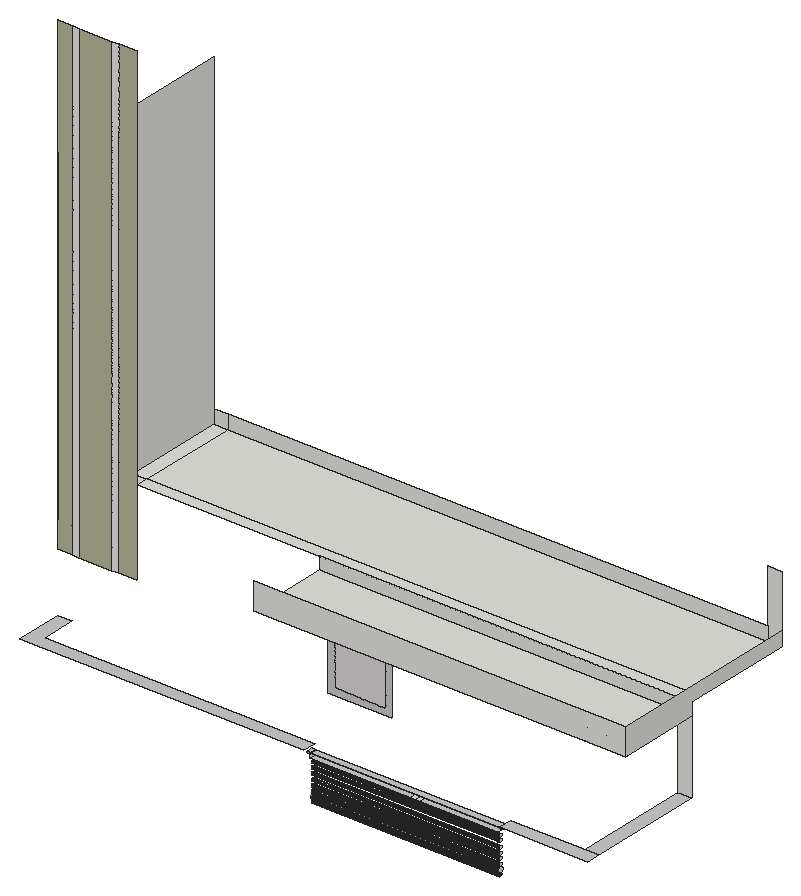
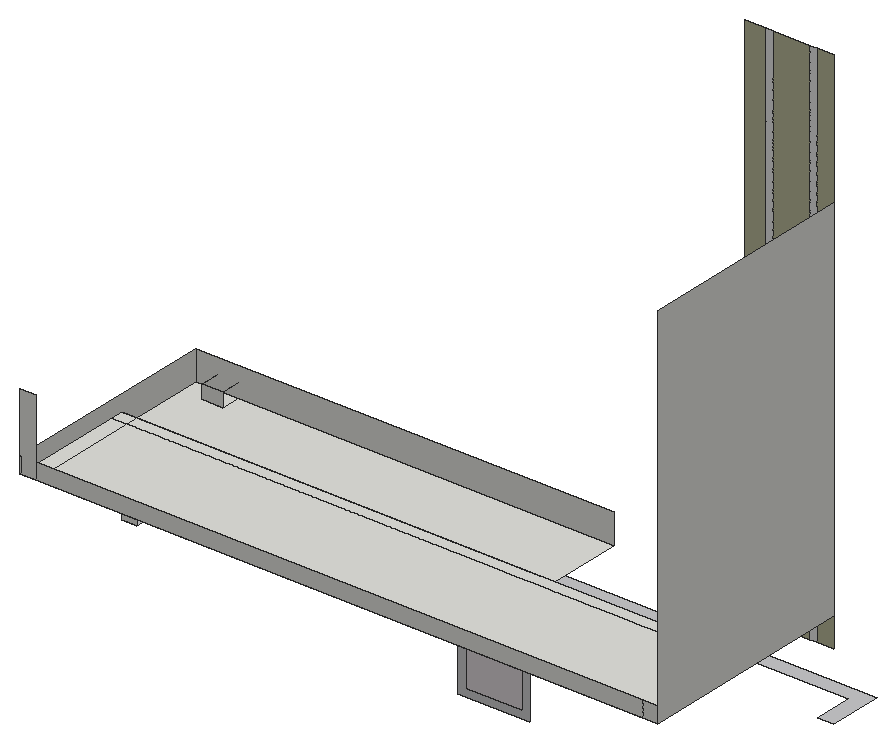
# SketchUp Ruby script. Lengths in inches.
U = 1.inch
M = Sketchup.active_model
def pt(a) = Geom::Point3d.new(a.map { |v| v * U })
def face(e, loops, mat)
  f = e.add_face(loops[0].map { |a| pt(a) })
  loops[1..].each { |l| e.add_face(l.map { |a| pt(a) }).erase! }
  f.material = f.back_material = mat if mat
  f
end
# faces: each face lists its corners as indices into pts; further lists are holes
def faces(e, pts, list, mat = nil) = list.each { |f| face(e, (f[0].is_a?(Array) ? f : [f]).map { |l| l.map { |i| pts[i] } }, mat) }
# xy, xz, yz: faces in a plane at the given z, y or x. An outline is a flat list of corners, or four numbers for a rectangle; further outlines are holes
def ring(l) = l.size == 4 ? [[l[0], l[1]], [l[2], l[1]], [l[2], l[3]], [l[0], l[3]]] : l.each_slice(2).to_a
def flat(e, list, mat, &to3) = list.each { |f| face(e, (f[0].is_a?(Array) ? f : [f]).map { |l| ring(l).map { |u, v| to3.(u, v) } }, mat) }
def xy(e, z, list, mat = nil) = flat(e, list, mat) { |x, y| [x, y, z] }
def xz(e, y, list, mat = nil) = flat(e, list, mat) { |x, z| [x, y, z] }
def yz(e, x, list, mat = nil) = flat(e, list, mat) { |y, z| [x, y, z] }
def lines(e, pts, list) = list.each { |a, b| e.add_line(pt(pts[a]), pt(pts[b])) }
# prism: a flat outline (further loops are holes) pulled along v
def prism(e, loops, v, mat = nil)
  f = face(e, loops, mat); d = Geom::Vector3d.new(v.map { |x| x * U })
  f.pushpull(f.normal.samedirection?(d) ? d.length : -d.length)
end
def box(e, o, s, mat = nil) = prism(e, [[o, [o[0] + s[0], o[1], o[2]], [o[0] + s[0], o[1] + s[1], o[2]], [o[0], o[1] + s[1], o[2]]]], [0, 0, s[2]], mat)
def at(x, y, z, deg = 0) = Geom::Transformation.translation(pt([x, y, z])) * Geom::Transformation.rotation(ORIGIN, Z_AXIS, deg.degrees)
def axes(o, x, y, z) = Geom::Transformation.new([*x, 0, *y, 0, *z, 0, *pt(o).to_a, 1])
def part(name) = M.definitions.add(name)
# library, detail: a bought-in or finely detailed component or shape, given as its bounding box
def library(name, o, s) = part(name).tap { |d| box(d.entities, o, s) }
def detail(e, o, s) = box(e.add_group.entities, o, s)
def put(e, d, t, mat = nil) = e.add_instance(d, t).tap { |i| i.material = mat if mat }
def group(e, t, mat = nil) = e.add_group.tap { |g| g.transformation = t; g.material = mat if mat }.entities
root = M.entities
M.materials.add("[Blinds Cellular White]").color = [217, 211, 213]
M.materials.add("[Concrete Form 4x8]").color = [167, 170, 168]
M.materials.add("[Polished Concrete New]").color = [200, 200, 203]
M.materials.add("[Polished Concrete Old]").color = [229, 229, 229]
M.materials.add("[Tile Linen]").color = [182, 181, 151]
xy(root,149.47,[[768.81,230.26,772.74,230.26,772.74,243.6875,764.33,243.6875,764.33,230.27],[754.67,230.27,764.33,243.6875],[754.67,243.6875,764.33,243.6875,764.33,243.85,754.67,243.86],[764.33,243.6875,772.74,243.6875,772.74,243.84,768.82,243.84,764.33,243.85]])
xy(root,149.47,[[562.43,230.1,562.43,243.6875,754.67,243.6875,754.67,230.27,764.33,230.27,768.81,230.26,772.74,230.26,772.74,243.6875,922.51,243.6875,922.51,230.1]],"[Polished Concrete New]")
xy(root,158.26,[[562.43,230.1,931.07,243.6875],[555.05,230.47,562.43,244.05]],"[Polished Concrete New]")
xy(root,163.5625,[[11.875,223.5,555.05,223.5,555.05,249.9,38.27,249.9,38.27,314.12,11.875,314.12],[931.07,223.5,1099.23,249.9],[1072.84,249.9,1099.23,472.99]],"[Polished Concrete New]")
xy(root,304.3125,[[386.67,314.12,386.67,472.99,1099.23,472.99,1099.23,314.12,1062.63,314.12,1062.63,346.6,1027.11,346.6,1027.11,314.12],[1027.11,314.12,1062.63,346.6]])
xy(root,328.125,[[11.875,472.99,38.27,494.96],[38.27,472.99,1072.84,494.96],[1072.84,472.99,1099.23,494.96],[11.875,494.96,38.27,688.57],[38.27,494.96,1072.84,688.57],
  [1072.84,494.96,1099.23,688.57]])
xz(root,230.1,[[562.43,158,931.07,158.26]])
xz(root,230.47,[[555.05,158,562.43,158.26]])
xz(root,314.12,[[386.67,304.3125,1099.23,354.875]])
xz(root,314.12,[[40.46,278.16,52.5,1185.41],[116.02,278.16,128.0625,1185.41]],"[Polished Concrete Old]")
xz(root,314.12,[[11.875,278.16,40.46,1185.41],[52.5,278.16,116.02,1185.41],[128.0625,278.16,163.125,1185.41]],"[Tile Linen]")
xz(root,346.6,[[1027.11,304.3125,1062.63,328.125]])
xz(root,472.99,[[1072.84,163.5625,1099.23,304.3125],[386.67,304.3125,1072.84,328.125],[1072.84,304.3125,1099.23,328.125]])
xz(root,472.99,[[414.74,111.09,512.86,284.96]],"[Blinds Cellular White]")
xz(root,472.99,[[[402.52,98.87,525.08,297.18],[414.74,111.09,512.86,284.96]]],"[Polished Concrete New]")
xz(root,688.57,[[11.875,328.125,38.27,354.875],[38.27,328.125,1072.84,354.875],[1072.84,328.125,1099.23,457.5]])
yz(root,11.875,[[314.12,328.125,688.57,958.5625]])
yz(root,562.43,[[230.1,149.47,230.47,158.26],[230.47,149.47,243.6875,158.26]])
yz(root,922.51,[[236.62,77.51,237.7,77.65,238.71,78.07,239.58,78.74,240.24,79.6,240.66,80.61,240.81,81.7,240.66,82.78,240.24,83.79,239.58,84.66,238.71,85.32,237.7,85.74,236.62,85.89,235.53,85.74,234.52,85.32,233.66,84.66,232.99,83.79,232.57,82.78,232.43,81.7,232.57,80.61,232.99,79.6,233.66,78.74,234.52,78.07,235.53,77.65],[236.71,89.28,237.35,89.36,237.93,89.61,238.4375,89.99,238.83,90.5,239.07,91.09,239.15,91.72,239.07,92.35,238.83,92.9375,238.4375,93.44,237.93,93.83,237.35,94.07,236.71,94.15,236.08,94.07,235.5,93.83,234.99,93.44,234.6,92.9375,234.36,92.35,234.28,91.72,234.36,91.09,234.6,90.5,234.99,89.99,235.5,89.61,236.08,89.36],[236.71,98.28,237.35,98.36,237.93,98.61,238.4375,98.99,238.83,99.5,239.07,100.09,239.15,100.72,239.07,101.35,238.83,101.9375,238.4375,102.44,237.93,102.83,237.35,103.07,236.71,103.15,236.08,103.07,235.5,102.83,234.99,102.44,234.6,101.9375,234.36,101.35,234.28,100.72,234.36,100.09,234.6,99.5,234.99,98.99,235.5,98.61,236.08,98.36],[236.71,108.15,237.35,108.24,237.93,108.48,238.4375,108.87,238.83,109.375,239.07,109.96,239.15,110.59,239.07,111.22,238.83,111.8125,238.4375,112.32,237.93,112.7,237.35,112.95,236.71,113.03,236.08,112.95,235.5,112.7,234.99,112.32,234.6,111.8125,234.36,111.22,234.28,110.59,234.36,109.96,234.6,109.375,234.99,108.87,235.5,108.48,236.08,108.24],[236.71,118.53,237.35,118.61,237.93,118.86,238.4375,119.24,238.83,119.75,239.07,120.34,239.15,120.97,239.07,121.6,238.83,122.1875,238.4375,122.69,237.93,123.08,237.35,123.32,236.71,123.4,236.08,123.32,235.5,123.08,234.99,122.69,234.6,122.1875,234.36,121.6,234.28,120.97,234.36,120.34,234.6,119.75,234.99,119.24,235.5,118.86,236.08,118.61],
  [236.71,129.34,237.35,129.43,237.93,129.67,238.4375,130.06,238.83,130.5625,239.07,131.15,239.15,131.78,239.07,132.41,238.83,133,238.4375,133.5,237.93,133.89,237.35,134.13,236.71,134.22,236.08,134.13,235.5,133.89,234.99,133.5,234.6,133,234.36,132.41,234.28,131.78,234.36,131.15,234.6,130.5625,234.99,130.06,235.5,129.67,236.08,129.43],[236.71,138.15,237.35,138.24,237.93,138.48,238.4375,138.87,238.83,139.375,239.07,139.96,239.15,140.59,239.07,141.22,238.83,141.8125,238.4375,142.32,237.93,142.7,237.35,142.95,236.71,143.03,236.08,142.95,235.5,142.7,234.99,142.32,234.6,141.8125,234.36,141.22,234.28,140.59,234.36,139.96,234.6,139.375,234.99,138.87,235.5,138.48,236.08,138.24]])
yz(root,1099.23,[[314.12,304.3125,472.99,304.3125,472.99,328.125,688.57,328.125,688.57,354.875,314.12,354.875]])
p = [[922.51,234.6,71.4375],[922.51,234.36,72.02],[562.43,234.36,72.02],[562.43,234.6,71.4375],[922.51,239.07,72.02],[922.51,238.83,71.4375],
  [562.43,238.83,71.4375],[562.43,239.07,72.02],[922.51,234.28,72.65],[562.43,234.28,72.65],[922.51,239.15,72.65],[562.43,239.15,72.65],
  [922.51,234.36,73.29],[562.43,234.36,73.29],[922.51,239.07,73.29],[562.43,239.07,73.29],[922.51,234.6,73.875],[562.43,234.6,73.875],
  [922.51,238.83,73.875],[562.43,238.83,73.875],[922.51,234.99,74.38],[562.43,234.99,74.38],[922.51,238.4375,74.38],[562.43,238.4375,74.38],
  [922.51,235.5,74.77],[562.43,235.5,74.77],[922.51,237.93,74.77],[562.43,237.93,74.77],[922.51,236.08,75.01],[562.43,236.08,75.01],
  [922.51,237.35,75.01],[562.43,237.35,75.01],[922.51,236.71,75.09],[562.43,236.71,75.09],[922.51,236.62,77.51],[922.51,235.53,77.65],
  [562.43,235.53,77.65],[562.43,236.62,77.51],[922.51,237.7,77.65],[562.43,237.7,77.65],[922.51,234.52,78.07],[562.43,234.52,78.07],
  [922.51,238.71,78.07],[562.43,238.71,78.07],[922.51,233.66,78.74],[562.43,233.66,78.74],[922.51,239.58,78.74],[562.43,239.58,78.74],
  [922.51,232.99,79.6],[562.43,232.99,79.6],[922.51,240.24,79.6],[562.43,240.24,79.6],[922.51,232.57,80.61],[562.43,232.57,80.61],
  [922.51,240.66,80.61],[562.43,240.66,80.61],[922.51,232.43,81.7],[562.43,232.43,81.7],[922.51,240.81,81.7],[562.43,240.81,81.7],
  [922.51,232.57,82.78],[562.43,232.57,82.78],[922.51,240.66,82.78],[562.43,240.66,82.78],[922.51,232.99,83.79],[562.43,232.99,83.79],
  [922.51,240.24,83.79],[562.43,240.24,83.79],[922.51,233.66,84.66],[562.43,233.66,84.66],[922.51,239.58,84.66],[562.43,239.58,84.66],
  [922.51,234.52,85.32],[562.43,234.52,85.32],[922.51,238.71,85.32],[562.43,238.71,85.32],[922.51,235.53,85.74],[562.43,235.53,85.74],
  [922.51,237.7,85.74],[562.43,237.7,85.74],[922.51,236.62,85.89],[562.43,236.62,85.89],[922.51,236.71,89.28],[922.51,236.08,89.36],
  [562.43,236.08,89.36],[562.43,236.71,89.28],[922.51,237.35,89.36],[562.43,237.35,89.36],[922.51,235.5,89.61],[562.43,235.5,89.61],
  [922.51,237.93,89.61],[562.43,237.93,89.61],[922.51,234.99,89.99],[562.43,234.99,89.99],[922.51,238.4375,89.99],[562.43,238.4375,89.99],
  [922.51,234.6,90.5],[562.43,234.6,90.5],[922.51,238.83,90.5],[562.43,238.83,90.5],[922.51,234.36,91.09],[562.43,234.36,91.09],
  [922.51,239.07,91.09],[562.43,239.07,91.09],[922.51,234.28,91.72],[562.43,234.28,91.72],[922.51,239.15,91.72],[562.43,239.15,91.72],
  [922.51,234.36,92.35],[562.43,234.36,92.35],[922.51,239.07,92.35],[562.43,239.07,92.35],[922.51,234.6,92.9375],[562.43,234.6,92.9375],
  [922.51,238.83,92.9375],[562.43,238.83,92.9375],[922.51,234.99,93.44],[562.43,234.99,93.44],[922.51,238.4375,93.44],[562.43,238.4375,93.44],
  [922.51,235.5,93.83],[562.43,235.5,93.83],[922.51,237.93,93.83],[562.43,237.93,93.83],[922.51,236.08,94.07],[562.43,236.08,94.07],
  [922.51,237.35,94.07],[562.43,237.35,94.07],[922.51,236.71,94.15],[562.43,236.71,94.15],[922.51,236.71,98.28],[922.51,236.08,98.36],
  [562.43,236.08,98.36],[562.43,236.71,98.28],[922.51,237.35,98.36],[562.43,237.35,98.36],[922.51,235.5,98.61],[562.43,235.5,98.61],
  [922.51,237.93,98.61],[562.43,237.93,98.61],[922.51,234.99,98.99],[562.43,234.99,98.99],[922.51,238.4375,98.99],[562.43,238.4375,98.99],
  [922.51,234.6,99.5],[562.43,234.6,99.5],[922.51,238.83,99.5],[562.43,238.83,99.5],[922.51,234.36,100.09],[562.43,234.36,100.09],
  [922.51,239.07,100.09],[562.43,239.07,100.09],[922.51,234.28,100.72],[562.43,234.28,100.72],[922.51,239.15,100.72],[562.43,239.15,100.72],
  [922.51,234.36,101.35],[562.43,234.36,101.35],[922.51,239.07,101.35],[562.43,239.07,101.35],[922.51,234.6,101.9375],[562.43,234.6,101.9375],
  [922.51,238.83,101.9375],[562.43,238.83,101.9375],[922.51,234.99,102.44],[562.43,234.99,102.44],[922.51,238.4375,102.44],[562.43,238.4375,102.44],
  [922.51,235.5,102.83],[562.43,235.5,102.83],[922.51,237.93,102.83],[562.43,237.93,102.83],[922.51,236.08,103.07],[562.43,236.08,103.07],
  [922.51,237.35,103.07],[562.43,237.35,103.07],[922.51,236.71,103.15],[562.43,236.71,103.15],[922.51,236.08,108.24],[922.51,235.5,108.48],
  [562.43,235.5,108.48],[562.43,236.08,108.24],[922.51,236.71,108.15],[562.43,236.71,108.15],[922.51,237.35,108.24],[562.43,237.35,108.24],
  [922.51,237.93,108.48],[562.43,237.93,108.48],[922.51,234.99,108.87],[562.43,234.99,108.87],[922.51,238.4375,108.87],[562.43,238.4375,108.87],
  [922.51,234.6,109.375],[562.43,234.6,109.375],[922.51,238.83,109.375],[562.43,238.83,109.375],[922.51,234.36,109.96],[562.43,234.36,109.96],
  [922.51,239.07,109.96],[562.43,239.07,109.96],[922.51,234.28,110.59],[562.43,234.28,110.59],[922.51,239.15,110.59],[562.43,239.15,110.59],
  [922.51,234.36,111.22],[562.43,234.36,111.22],[922.51,239.07,111.22],[562.43,239.07,111.22],[922.51,234.6,111.8125],[562.43,234.6,111.8125],
  [922.51,238.83,111.8125],[562.43,238.83,111.8125],[922.51,234.99,112.32],[562.43,234.99,112.32],[922.51,238.4375,112.32],[562.43,238.4375,112.32],
  [922.51,235.5,112.7],[562.43,235.5,112.7],[922.51,237.93,112.7],[562.43,237.93,112.7],[922.51,236.08,112.95],[562.43,236.08,112.95],
  [922.51,237.35,112.95],[562.43,237.35,112.95],[922.51,236.71,113.03],[562.43,236.71,113.03],[922.51,236.71,118.53],[922.51,236.08,118.61],
  [562.43,236.08,118.61],[562.43,236.71,118.53],[922.51,237.35,118.61],[562.43,237.35,118.61],[922.51,235.5,118.86],[562.43,235.5,118.86],
  [922.51,237.93,118.86],[562.43,237.93,118.86],[922.51,234.99,119.24],[562.43,234.99,119.24],[922.51,238.4375,119.24],[562.43,238.4375,119.24],
  [922.51,234.6,119.75],[562.43,234.6,119.75],[922.51,238.83,119.75],[562.43,238.83,119.75],[922.51,234.36,120.34],[562.43,234.36,120.34],
  [922.51,239.07,120.34],[562.43,239.07,120.34],[922.51,234.28,120.97],[562.43,234.28,120.97],[922.51,239.15,120.97],[562.43,239.15,120.97],
  [922.51,234.36,121.6],[562.43,234.36,121.6],[922.51,239.07,121.6],[562.43,239.07,121.6],[922.51,234.6,122.1875],[562.43,234.6,122.1875],
  [922.51,238.83,122.1875],[562.43,238.83,122.1875],[922.51,234.99,122.69],[562.43,234.99,122.69],[922.51,238.4375,122.69],[562.43,238.4375,122.69],
  [922.51,235.5,123.08],[562.43,235.5,123.08],[922.51,237.93,123.08],[562.43,237.93,123.08],[922.51,236.08,123.32],[562.43,236.08,123.32],
  [922.51,237.35,123.32],[562.43,237.35,123.32],[922.51,236.71,123.4],[562.43,236.71,123.4],[922.51,236.71,129.34],[922.51,236.08,129.43],
  [562.43,236.08,129.43],[562.43,236.71,129.34],[922.51,237.35,129.43],[562.43,237.35,129.43],[922.51,235.5,129.67],[562.43,235.5,129.67],
  [922.51,237.93,129.67],[562.43,237.93,129.67],[922.51,234.99,130.06],[562.43,234.99,130.06],[922.51,238.4375,130.06],[562.43,238.4375,130.06],
  [922.51,234.6,130.5625],[562.43,234.6,130.5625],[922.51,238.83,130.5625],[562.43,238.83,130.5625],[922.51,234.36,131.15],[562.43,234.36,131.15],
  [922.51,239.07,131.15],[562.43,239.07,131.15],[922.51,234.28,131.78],[562.43,234.28,131.78],[922.51,239.15,131.78],[562.43,239.15,131.78],
  [922.51,234.36,132.41],[562.43,234.36,132.41],[922.51,239.07,132.41],[562.43,239.07,132.41],[922.51,234.6,133],[562.43,234.6,133],
  [922.51,238.83,133],[562.43,238.83,133],[922.51,234.99,133.5],[562.43,234.99,133.5],[922.51,238.4375,133.5],[562.43,238.4375,133.5],
  [922.51,235.5,133.89],[562.43,235.5,133.89],[922.51,237.93,133.89],[562.43,237.93,133.89],[922.51,236.08,134.13],[562.43,236.08,134.13],
  [922.51,237.35,134.13],[562.43,237.35,134.13],[922.51,236.71,134.22],[562.43,236.71,134.22],[922.51,236.08,138.24],[922.51,235.5,138.48],
  [562.43,235.5,138.48],[562.43,236.08,138.24],[922.51,236.71,138.15],[562.43,236.71,138.15],[922.51,237.35,138.24],[562.43,237.35,138.24],
  [922.51,237.93,138.48],[562.43,237.93,138.48],[922.51,234.99,138.87],[562.43,234.99,138.87],[922.51,238.4375,138.87],[562.43,238.4375,138.87],
  [922.51,234.6,139.375],[562.43,234.6,139.375],[922.51,238.83,139.375],[562.43,238.83,139.375],[922.51,234.36,139.96],[562.43,234.36,139.96],
  [922.51,239.07,139.96],[562.43,239.07,139.96],[922.51,234.28,140.59],[562.43,234.28,140.59],[922.51,239.15,140.59],[562.43,239.15,140.59],
  [922.51,234.36,141.22],[562.43,234.36,141.22],[922.51,239.07,141.22],[562.43,239.07,141.22],[922.51,234.6,141.8125],[562.43,234.6,141.8125],
  [922.51,238.83,141.8125],[562.43,238.83,141.8125],[922.51,234.99,142.32],[562.43,234.99,142.32],[922.51,238.4375,142.32],[562.43,238.4375,142.32],
  [922.51,235.5,142.7],[562.43,235.5,142.7],[922.51,237.93,142.7],[562.43,237.93,142.7],[922.51,236.08,142.95],[562.43,236.08,142.95],
  [922.51,237.35,142.95],[562.43,237.35,142.95],[922.51,236.71,143.03],[562.43,236.71,143.03],[1062.63,346.6,328.125],[1062.63,314.12,328.125],
  [1027.11,346.6,328.125],[1027.11,314.12,328.125],[38.27,472.99,328.125],[38.27,314.12,328.125]]
faces(root,p,[[0,1,2,3],[4,5,6,7],[1,8,9,2],[10,4,7,11],[8,12,13,9],[14,10,11,15],[12,16,17,13],[18,14,15,19],
  [16,20,21,17],[22,18,19,23],[20,24,25,21],[26,22,23,27],[24,28,29,25],[30,26,27,31],[28,32,33,29],[32,30,31,33],
  [82,83,84,85],[86,82,85,87],[83,88,89,84],[90,86,87,91],[88,92,93,89],[94,90,91,95],[92,96,97,93],[98,94,95,99],
  [96,100,101,97],[102,98,99,103],[100,104,105,101],[106,102,103,107],[104,108,109,105],[110,106,107,111],[108,112,113,109],[114,110,111,115],
  [112,116,117,113],[118,114,115,119],[116,120,121,117],[122,118,119,123],[120,124,125,121],[126,122,123,127],[124,128,129,125],[128,126,127,129],
  [130,131,132,133],[134,130,133,135],[131,136,137,132],[138,134,135,139],[136,140,141,137],[142,138,139,143],[140,144,145,141],[146,142,143,147],
  [144,148,149,145],[150,146,147,151],[148,152,153,149],[154,150,151,155],[152,156,157,153],[158,154,155,159],[156,160,161,157],[162,158,159,163],
  [160,164,165,161],[166,162,163,167],[164,168,169,165],[170,166,167,171],[168,172,173,169],[174,170,171,175],[172,176,177,173],[176,174,175,177],
  [178,179,180,181],[182,178,181,183],[184,182,183,185],[186,184,185,187],[179,188,189,180],[190,186,187,191],[188,192,193,189],[194,190,191,195],
  [192,196,197,193],[198,194,195,199],[196,200,201,197],[202,198,199,203],[200,204,205,201],[206,202,203,207],[204,208,209,205],[210,206,207,211],
  [208,212,213,209],[214,210,211,215],[212,216,217,213],[218,214,215,219],[216,220,221,217],[222,218,219,223],[220,224,225,221],[224,222,223,225],
  [226,227,228,229],[230,226,229,231],[227,232,233,228],[234,230,231,235],[232,236,237,233],[238,234,235,239],[236,240,241,237],[242,238,239,243],
  [240,244,245,241],[246,242,243,247],[244,248,249,245],[250,246,247,251],[248,252,253,249],[254,250,251,255],[252,256,257,253],[258,254,255,259],
  [256,260,261,257],[262,258,259,263],[260,264,265,261],[266,262,263,267],[264,268,269,265],[270,266,267,271],[268,272,273,269],[272,270,271,273],
  [274,275,276,277],[278,274,277,279],[275,280,281,276],[282,278,279,283],[280,284,285,281],[286,282,283,287],[284,288,289,285],[290,286,287,291],
  [288,292,293,289],[294,290,291,295],[292,296,297,293],[298,294,295,299],[296,300,301,297],[302,298,299,303],[300,304,305,301],[306,302,303,307],
  [304,308,309,305],[310,306,307,311],[308,312,313,309],[314,310,311,315],[312,316,317,313],[318,314,315,319],[316,320,321,317],[320,318,319,321],
  [322,323,324,325],[326,322,325,327],[328,326,327,329],[330,328,329,331],[323,332,333,324],[334,330,331,335],[332,336,337,333],[338,334,335,339],
  [336,340,341,337],[342,338,339,343],[340,344,345,341],[346,342,343,347],[344,348,349,345],[350,346,347,351],[348,352,353,349],[354,350,351,355],
  [352,356,357,353],[358,354,355,359],[356,360,361,357],[362,358,359,363],[360,364,365,361],[366,362,363,367],[364,368,369,365],[368,366,367,369]],"[Polished Concrete Old]")
faces(root,p,[[34,35,36,37],[38,34,37,39],[35,40,41,36],[42,38,39,43],[40,44,45,41],[46,42,43,47],[44,48,49,45],[50,46,47,51],
  [48,52,53,49],[54,50,51,55],[52,56,57,53],[58,54,55,59],[56,60,61,57],[62,58,59,63],[60,64,65,61],[66,62,63,67],
  [64,68,69,65],[70,66,67,71],[68,72,73,69],[74,70,71,75],[72,76,77,73],[78,74,75,79],[76,80,81,77],[80,78,79,81]],"[Concrete Form 4x8]")
lines(root,p,[[370,371],[372,373],[374,375]])
